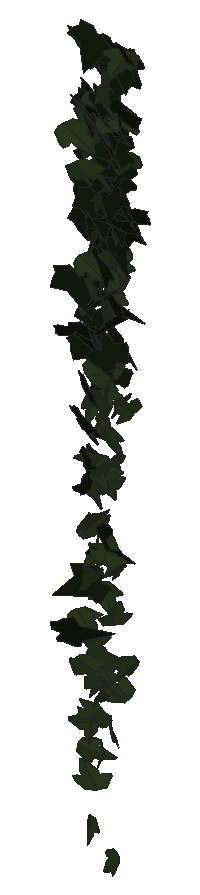
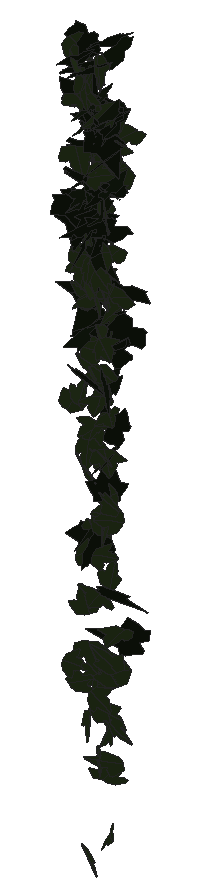
# SketchUp Ruby script. Lengths in inches.
U = 1.inch
M = Sketchup.active_model
def pt(a) = Geom::Point3d.new(a.map { |v| v * U })
def face(e, loops, mat)
  f = e.add_face(loops[0].map { |a| pt(a) })
  loops[1..].each { |l| e.add_face(l.map { |a| pt(a) }).erase! }
  f.material = f.back_material = mat if mat
  f
end
# faces: each face lists its corners as indices into pts; further lists are holes
def faces(e, pts, list, mat = nil) = list.each { |f| face(e, (f[0].is_a?(Array) ? f : [f]).map { |l| l.map { |i| pts[i] } }, mat) }
# xy, xz, yz: faces in a plane at the given z, y or x. An outline is a flat list of corners, or four numbers for a rectangle; further outlines are holes
def ring(l) = l.size == 4 ? [[l[0], l[1]], [l[2], l[1]], [l[2], l[3]], [l[0], l[3]]] : l.each_slice(2).to_a
def flat(e, list, mat, &to3) = list.each { |f| face(e, (f[0].is_a?(Array) ? f : [f]).map { |l| ring(l).map { |u, v| to3.(u, v) } }, mat) }
def xy(e, z, list, mat = nil) = flat(e, list, mat) { |x, y| [x, y, z] }
def xz(e, y, list, mat = nil) = flat(e, list, mat) { |x, z| [x, y, z] }
def yz(e, x, list, mat = nil) = flat(e, list, mat) { |y, z| [x, y, z] }
def lines(e, pts, list) = list.each { |a, b| e.add_line(pt(pts[a]), pt(pts[b])) }
# prism: a flat outline (further loops are holes) pulled along v
def prism(e, loops, v, mat = nil)
  f = face(e, loops, mat); d = Geom::Vector3d.new(v.map { |x| x * U })
  f.pushpull(f.normal.samedirection?(d) ? d.length : -d.length)
end
def box(e, o, s, mat = nil) = prism(e, [[o, [o[0] + s[0], o[1], o[2]], [o[0] + s[0], o[1] + s[1], o[2]], [o[0], o[1] + s[1], o[2]]]], [0, 0, s[2]], mat)
def at(x, y, z, deg = 0) = Geom::Transformation.translation(pt([x, y, z])) * Geom::Transformation.rotation(ORIGIN, Z_AXIS, deg.degrees)
def axes(o, x, y, z) = Geom::Transformation.new([*x, 0, *y, 0, *z, 0, *pt(o).to_a, 1])
def part(name) = M.definitions.add(name)
# library, detail: a bought-in or finely detailed component or shape, given as its bounding box
def library(name, o, s) = part(name).tap { |d| box(d.entities, o, s) }
def detail(e, o, s) = box(e.add_group.entities, o, s)
def put(e, d, t, mat = nil) = e.add_instance(d, t).tap { |i| i.material = mat if mat }
def group(e, t, mat = nil) = e.add_group.tap { |g| g.transformation = t; g.material = mat if mat }.entities
root = M.entities
M.materials.add("1026 AP 7946 SUNNY SIDE UP").color = [254, 231, 186]
M.materials.add("efeu1").color = [18, 25, 13]
M.materials.add("efeu2").color = [43, 57, 29]
c1 = part("ivyleaf_9")
p = [[1.54,2.16,1.25],[1.36,2.04,1.19],[-0.21,0.99,0.68],[-0.71,1.11,0.82],[-0.85,0.86,0.67],[-0.8,0.17,0.21],
  [-0.9,-0.01,0.1],[-0.67,-0.16,-0.02],[-0.08,-0.08,-0.05],[-0.03,-0.6,-0.4],[0.65,-0.88,-0.66],[0.83,-0.6,-0.49],
  [1.29,-0.42,-0.43],[1.8125,-0.07,-0.26],[1.21,0.44,0.15]]
faces(c1.entities,p,[[0,1,2,3,4,5,6,7,8,9,10,11,12,13,14]],"efeu1")
c2 = part("ivyleaf_10")
p = [[0,0.5,-0.03],[-0.0625,2.02,-0.43],[-0.19,2.01,-0.46],[-0.54,1.05,-0.29],[-0.52,0.625,-0.18],[-0.83,0.76,-0.28],
  [-1.16,0.64,-0.33],[-1.15,0.33,-0.24],[-0.77,-0.39,0.02],[-0.3,-0.51,0.16],[0.04,-0.48,0.23],[-0.02,2.01,-0.4375],
  [-0.06,2.01,-0.43],[0.04,-0.49,0.23],[0.67,-0.49,0.14],[1.38,0.36,-0.2],[1.375,0.51,-0.24],[0.81,0.65,-0.19],
  [0.62,0.59,-0.15],[0.6,1.09,-0.28],[0.5,1.23,-0.31]]
faces(c2.entities,p,[[0,1,2,3,4,5,6,7,8,9,10],[11,12,0,13,14,15,16,17,18,19,20]],"efeu2")
put(root,c1,axes([109.1,212.42,255.3],[-0.38815,-0.01415,0.07817],[-0.11542,-0.0364,-0.25296],[0.03792,-0.25569,0.03015]),"1026 AP 7946 SUNNY SIDE UP")
put(root,c2,axes([108.73,212.32,254.46],[0.18641,0.16961,0.10073],[0.10772,0.06995,-0.21225],[-0.28757,0.13615,-0.01421]),"1026 AP 7946 SUNNY SIDE UP")
put(root,c1,axes([108.57,212,254.15],[0.14545,0.03079,0.24435],[0.37278,0.02041,-0.09793],[-0.04766,0.25361,-0.02027]),"1026 AP 7946 SUNNY SIDE UP")
put(root,c2,axes([109.09,212.18,252.21],[0.12202,-0.07291,-0.21039],[-0.26996,0.11112,-0.10765],[0.20728,0.18765,-0.01635]),"1026 AP 7946 SUNNY SIDE UP")
put(root,c1,axes([108.75,212.23,262.23],[-0.21159,-0.16583,-0.18391],[0.21642,0.11526,-0.21765],[0.31483,-0.19068,0.02602]),"1026 AP 7946 SUNNY SIDE UP")
put(root,c2,axes([108.97,212.4,265.37],[-0.21301,-0.21353,0.03478],[-0.01266,-0.03626,-0.26041],[0.34,-0.13513,0.01209]),"1026 AP 7946 SUNNY SIDE UP")
put(root,c1,axes([108.78,211.94,261.17],[0.33078,0.13445,0.03505],[0.05691,0.00503,-0.2567],[-0.21022,0.21292,-0.01433]),"1026 AP 7946 SUNNY SIDE UP")
put(root,c2,axes([108.76,212.56,253.77],[-0.23079,-0.03638,0.15843],[0.23189,0.04469,0.15594],[-0.09019,0.20799,-0.00448]),"1026 AP 7946 SUNNY SIDE UP")
put(root,c2,axes([108.93,212.64,261.03],[-0.07149,-0.19972,0.1003],[0.04657,-0.10506,-0.20599],[0.34704,-0.02705,0.0483]),"1026 AP 7946 SUNNY SIDE UP")
put(root,c2,axes([108.87,212.35,253.33],[-0.22474,-0.15958,0.07883],[0.06279,0.06792,0.22058],[-0.27174,0.14768,-0.01422]),"1026 AP 7946 SUNNY SIDE UP")
put(root,c2,axes([108.96,212.1875,261.63],[-0.02158,0.04342,0.26265],[-0.10296,0.24615,-0.04542],[-0.39301,-0.06687,-0.00253]),"1026 AP 7946 SUNNY SIDE UP")
put(root,c1,axes([108.78,212.55,264.56],[-0.03434,-0.15433,0.22207],[0.06502,-0.21649,-0.15601],[0.41289,0.02126,0.04303]),"1026 AP 7946 SUNNY SIDE UP")
put(root,c2,axes([108.74,211.99,265.625],[0.20152,0.17099,0.17042],[0.1784,0.11998,-0.2189],[-0.32761,0.17052,-0.01437]),"1026 AP 7946 SUNNY SIDE UP")
put(root,c1,axes([108.71,212.29,267.6],[0.23756,-0.22005,0.04774],[0.02223,-0.04792,-0.27481],[0.3533,0.15098,-0.01481]),"1026 AP 7946 SUNNY SIDE UP")
put(root,c1,axes([109.13,212.34,260.06],[-0.05281,0.00819,-0.2693],[-0.35441,0.13288,0.0349],[0.20875,0.22767,-0.00889]),"1026 AP 7946 SUNNY SIDE UP")
put(root,c1,axes([109.09,212.43,265.58],[0.02018,0.23184,-0.11035],[-0.02405,-0.10768,-0.23968],[-0.40173,0.01809,0.0088]),"1026 AP 7946 SUNNY SIDE UP")
put(root,c2,axes([108.95,212.42,259.36],[0.09128,0.19116,-0.08595],[-0.03412,-0.08173,-0.20627],[-0.32688,0.06191,-0.00247]),"1026 AP 7946 SUNNY SIDE UP")
put(root,c2,axes([108.7,212.33,262.07],[0.1886,0.07448,0.21711],[0.31936,0.06243,-0.14173],[-0.14526,0.23394,-0.0297]),"1026 AP 7946 SUNNY SIDE UP")
put(root,c2,axes([108.95,212.4,249.82],[-0.01188,0.16367,-0.1463],[0.00065,-0.14302,-0.16956],[-0.34169,-0.00596,0.00477]),"1026 AP 7946 SUNNY SIDE UP")
put(root,c1,axes([108.9,212.52,266.07],[-0.06238,-0.24185,0.05581],[0.00398,-0.05664,-0.25254],[0.39017,-0.03809,0.0115]),"1026 AP 7946 SUNNY SIDE UP")
put(root,c2,axes([109.16,212.64,264.79],[0.01493,0.02693,-0.25317],[-0.21949,-0.20258,-0.02959],[-0.32112,0.13972,0.00846]),"1026 AP 7946 SUNNY SIDE UP")
put(root,c2,axes([109.1,212.65,253.02],[-0.05691,-0.17814,0.1263],[-0.02331,-0.12299,-0.18779],[0.34013,-0.03823,0.00826]),"1026 AP 7946 SUNNY SIDE UP")
put(root,c1,axes([108.83,212.65,266.18],[0.04476,-0.19415,0.17082],[0.10756,-0.15608,-0.19995],[0.38797,0.06567,0.03573]),"1026 AP 7946 SUNNY SIDE UP")
put(root,c2,axes([109.06,212.59,262.52],[-0.07905,-0.19679,0.13343],[0.04578,-0.13771,-0.20297],[0.36858,-0.0251,0.05383]),"1026 AP 7946 SUNNY SIDE UP")
put(root,c2,axes([108.8,212.52,257.36],[0.09621,-0.0488,-0.21654],[0.29213,-0.09864,0.07884],[-0.17174,-0.19514,0.01279]),"1026 AP 7946 SUNNY SIDE UP")
put(root,c1,axes([108.8,212.31,265.98],[0.21385,-0.19938,0.12808],[0.09432,-0.11078,-0.249],[0.35819,0.1482,-0.0109]),"1026 AP 7946 SUNNY SIDE UP")
put(root,c2,axes([109.01,212.57,263.93],[0.2113,-0.17684,0.10631],[0.08467,-0.08981,-0.22908],[0.31143,0.1444,-0.00985]),"1026 AP 7946 SUNNY SIDE UP")
put(root,c2,axes([109.2,212.16,261.99],[-0.04608,0.16708,-0.20215],[-0.1195,0.1841,0.17342],[0.38842,0.07646,0.02937]),"1026 AP 7946 SUNNY SIDE UP")
put(root,c2,axes([109.29,212.22,252.48],[-0.23547,-0.01911,0.18146],[-0.25383,-0.08069,-0.15078],[0.11526,-0.21675,0.03868]),"1026 AP 7946 SUNNY SIDE UP")
put(root,c2,axes([109.09,212.32,263.98],[0.08737,-0.24272,-0.07457],[0.01003,0.07402,-0.25509],[0.39753,0.05148,0.02283]),"1026 AP 7946 SUNNY SIDE UP")
put(root,c1,axes([109.18,212.59,263.11],[-0.22209,0.16617,-0.14295],[0.12399,-0.11602,-0.22497],[-0.31804,-0.16127,0.01212]),"1026 AP 7946 SUNNY SIDE UP")
put(root,c2,axes([108.96,212.32,257.51],[-0.21131,0.1088,-0.13734],[0.14687,-0.09687,-0.17818],[-0.22814,-0.16314,0.0125]),"1026 AP 7946 SUNNY SIDE UP")
put(root,c1,axes([109.04,212.3,257.48],[0.2081,0.14691,0.18135],[-0.22047,-0.10776,0.20157],[0.28398,-0.19131,0.02359]),"1026 AP 7946 SUNNY SIDE UP")
put(root,c2,axes([108.93,212.29,266.15],[-0.11879,-0.11934,-0.25786],[0.27281,0.18114,-0.14225],[0.3389,-0.18764,0.02413]),"1026 AP 7946 SUNNY SIDE UP")
put(root,c1,axes([108.78,212.24,258.97],[0.2698,-0.05383,-0.20882],[0.31725,-0.02766,0.18363],[-0.08828,-0.26389,0.02173]),"1026 AP 7946 SUNNY SIDE UP")
put(root,c2,axes([109.12,212.1875,252.06],[0.01524,-0.06895,-0.22623],[0.00945,0.2194,-0.06954],[0.36121,-0.00283,0.01136]),"1026 AP 7946 SUNNY SIDE UP")
put(root,c2,axes([109.1,212.22,255.43],[-0.06568,-0.19125,-0.12492],[-0.05705,-0.11495,0.20077],[-0.35055,0.05454,-0.00927]),"1026 AP 7946 SUNNY SIDE UP")
put(root,c1,axes([109.11,212.57,262.99],[-0.00649,0.04166,0.26319],[-0.19141,-0.22554,0.03458],[0.35878,-0.11957,0.02321]),"1026 AP 7946 SUNNY SIDE UP")
put(root,c2,axes([108.84,212.38,251.48],[-0.05062,-0.03342,-0.21837],[0.33673,0.00528,-0.03436],[0.0162,-0.21414,0.03194]),"1026 AP 7946 SUNNY SIDE UP")
put(root,c1,axes([108.8,212.18,260.78],[0.36176,-0.06074,0.10227],[0.14407,-0.0423,-0.24482],[0.11358,0.24711,-0.0152]),"1026 AP 7946 SUNNY SIDE UP")
put(root,c2,axes([109.13,212.51,267.29],[0.05166,-0.25355,-0.08],[0.01371,0.0778,-0.26229],[0.41608,0.02892,0.01857]),"1026 AP 7946 SUNNY SIDE UP")
put(root,c1,axes([109.05,212.03,259.98],[0.2795,-0.12137,-0.15354],[-0.20339,0.07335,-0.22106],[0.22242,0.2196,-0.00921]),"1026 AP 7946 SUNNY SIDE UP")
put(root,c1,axes([108.96,212.2,260.86],[0.0944,-0.22294,-0.15102],[0.00557,0.14964,-0.2341],[0.41842,0.0483,0.03719]),"1026 AP 7946 SUNNY SIDE UP")
put(root,c2,axes([108.93,212.1,264.78],[-0.27511,-0.02265,-0.2007],[0.3077,-0.00546,-0.18055],[0.0174,-0.2617,0.01959]),"1026 AP 7946 SUNNY SIDE UP")
put(root,c1,axes([108.99,212.33,264.43],[0.01334,-0.1861,-0.17521],[0.03684,0.16897,-0.18946],[0.39358,-0.00951,0.02367]),"1026 AP 7946 SUNNY SIDE UP")
put(root,c2,axes([109.1,212.01,256.7],[0.03317,-0.11659,0.25117],[-0.01919,0.24456,0.12267],[-0.42545,-0.02012,0.01405]),"1026 AP 7946 SUNNY SIDE UP")
put(root,c2,axes([109.22,212.21,258.25],[-0.25452,-0.13901,0.03922],[-0.02758,-0.03901,-0.21926],[0.22528,-0.16183,0.01746]),"1026 AP 7946 SUNNY SIDE UP")
put(root,c1,axes([108.87,212.42,263.65],[0.13034,-0.11315,-0.27031],[0.1436,0.26876,-0.08832],[0.42477,-0.05614,0.1128]),"1026 AP 7946 SUNNY SIDE UP")
put(root,c2,axes([109.23,212.14,250.91],[0.27143,0.13233,0.0767],[-0.11265,-0.02713,0.22288],[0.20985,-0.18573,0.02043]),"1026 AP 7946 SUNNY SIDE UP")
put(root,c1,axes([109.12,212.33,267.72],[-0.15424,-0.24288,0.06762],[-0.01758,-0.06765,-0.26983],[0.39578,-0.09766,0.01437]),"1026 AP 7946 SUNNY SIDE UP")
put(root,c2,axes([109.34,212.51,260.72],[-0.11031,-0.03293,0.23146],[-0.16658,-0.20346,-0.06594],[0.31615,-0.1187,0.04602]),"1026 AP 7946 SUNNY SIDE UP")
put(root,c1,axes([109.28,212.61,264.8],[-0.01787,-0.24776,-0.01424],[0.0105,-0.01273,0.25533],[-0.38993,0.01101,0.00753]),"1026 AP 7946 SUNNY SIDE UP")
put(root,c2,axes([109.2,212.375,261.09],[0.1178,-0.2316,0.0199],[-0.0008,-0.02184,-0.25078],[0.36561,0.07457,-0.00696]),"1026 AP 7946 SUNNY SIDE UP")
put(root,c1,axes([109.05,212.1875,258.3125],[0.20173,-0.19112,-0.08823],[-0.08317,0.06629,-0.23665],[0.31791,0.13862,-0.00593]),"1026 AP 7946 SUNNY SIDE UP")
put(root,c2,axes([109.27,212.22,262.15],[0.09097,-0.2529,-0.10954],[-0.05717,0.09916,-0.26638],[0.42669,0.0672,-0.01233]),"1026 AP 7946 SUNNY SIDE UP")
put(root,c2,axes([108.98,212.12,253.57],[-0.24192,-0.02677,-0.19972],[0.307,-0.0071,-0.15878],[0.01738,-0.24728,0.02471]),"1026 AP 7946 SUNNY SIDE UP")
put(root,c1,axes([109.1,212.34,261.45],[-0.04941,-0.23988,0.01052],[0.0024,-0.01188,-0.24928],[0.37761,-0.03131,0.00296]),"1026 AP 7946 SUNNY SIDE UP")
put(root,c2,axes([109.24,212.375,256.03],[-0.06052,-0.07486,0.21873],[0.00215,-0.21589,-0.07926],[0.35461,-0.01146,0.03781]),"1026 AP 7946 SUNNY SIDE UP")
put(root,c2,axes([109.21,212.33,256.63],[-0.06336,-0.1851,-0.13479],[-0.06214,-0.12404,0.19416],[-0.35,0.05553,-0.01007]),"1026 AP 7946 SUNNY SIDE UP")
put(root,c2,axes([109.03,212.49,263.04],[-0.23081,0.09377,-0.20178],[0.23223,-0.13107,-0.17895],[-0.25134,-0.20721,0.01994]),"1026 AP 7946 SUNNY SIDE UP")
put(root,c2,axes([109.28,212.31,251.52],[0.05424,-0.13626,-0.18309],[-0.06045,0.17275,-0.14376],[0.34593,0.05156,0.00359]),"1026 AP 7946 SUNNY SIDE UP")
put(root,c2,axes([109.22,212.45,259.03],[0.04481,0.11391,-0.19473],[-0.04984,-0.18717,-0.12179],[-0.3443,0.04192,-0.00771]),"1026 AP 7946 SUNNY SIDE UP")
put(root,c2,axes([109.12,212.38,256.47],[-0.13424,0.10621,0.1911],[0.19681,-0.13628,0.13939],[0.27145,0.15134,-0.00656]),"1026 AP 7946 SUNNY SIDE UP")
put(root,c1,axes([109.01,212.5625,263.98],[0.16505,-0.19349,0.11075],[0.07694,-0.097,-0.22732],[0.3403,0.11578,-0.00232]),"1026 AP 7946 SUNNY SIDE UP")
put(root,c2,axes([109.13,211.99,262.78],[0.16347,0.16372,0.14106],[0.0869,0.12539,-0.19831],[-0.32318,0.11653,0.01803]),"1026 AP 7946 SUNNY SIDE UP")
put(root,c2,axes([109.18,212.43,259.61],[0.19646,0.17664,0.02335],[0.03232,0.01196,-0.22259],[-0.27795,0.12624,-0.00938]),"1026 AP 7946 SUNNY SIDE UP")
put(root,c1,axes([108.9375,212.3,265.94],[0.29981,-0.11614,0.1605],[0.18608,-0.10488,-0.22939],[0.2434,0.22323,-0.02232]),"1026 AP 7946 SUNNY SIDE UP")
put(root,c2,axes([109.32,212.4,262],[0.09849,-0.21173,-0.07683],[-0.03496,0.06994,-0.22705],[0.35061,0.06645,-0.00106]),"1026 AP 7946 SUNNY SIDE UP")
put(root,c2,axes([109.27,211.99,256.78],[0.04966,-0.12151,0.2227],[-0.04128,0.21576,0.12974],[-0.38869,-0.03844,0.01467]),"1026 AP 7946 SUNNY SIDE UP")
put(root,c1,axes([109.18,212.44,263.78],[-0.00235,-0.13896,-0.21718],[0.01837,0.20976,-0.14184],[0.39556,-0.01057,0.0053]),"1026 AP 7946 SUNNY SIDE UP")
put(root,c1,axes([109.15,212.57,262.94],[0.13246,-0.22421,-0.04493],[-0.01752,0.04104,-0.24647],[0.35836,0.08488,0.00456]),"1026 AP 7946 SUNNY SIDE UP")
put(root,c2,axes([109.34,212.54,263.24],[0.04606,-0.23911,0.00205],[-0.00028,-0.00339,-0.24819],[0.37602,0.02929,-0.00044]),"1026 AP 7946 SUNNY SIDE UP")
put(root,c2,axes([109.25,212.1,261.02],[-0.20282,0.16408,-0.0839],[0.06941,-0.07001,-0.21526],[-0.28022,-0.1361,0.00741]),"1026 AP 7946 SUNNY SIDE UP")
put(root,c2,axes([109.33,212.15,263.5],[0.1065,-0.25129,0.07105],[0.02769,-0.06816,-0.26852],[0.40941,0.06998,-0.00032]),"1026 AP 7946 SUNNY SIDE UP")
put(root,c2,axes([109.46,212.28,263.0625],[-0.28333,0.12914,0.09329],[-0.13641,0.03235,-0.22702],[-0.20634,-0.19872,0.02198]),"1026 AP 7946 SUNNY SIDE UP")
put(root,c1,axes([109.33,212.72,267.14],[-0.16586,-0.21841,0.0802],[-0.01311,-0.08324,-0.24877],[0.36501,-0.10223,0.02751]),"1026 AP 7946 SUNNY SIDE UP")
put(root,c2,axes([109.1875,212.45,255.17],[0.32125,0.02493,0.11475],[0.17766,-0.01384,-0.21065],[-0.0239,0.23222,-0.0235]),"1026 AP 7946 SUNNY SIDE UP")
put(root,c1,axes([109.21,212.27,266.43],[0.27385,-0.16914,-0.13276],[-0.09838,0.11716,-0.24669],[0.3186,0.18156,0.03794]),"1026 AP 7946 SUNNY SIDE UP")
put(root,c2,axes([109.36,212.55,262.25],[0.07443,-0.19876,0.10275],[0.05186,-0.09574,-0.21085],[0.34662,0.057,0.00948]),"1026 AP 7946 SUNNY SIDE UP")
put(root,c2,axes([109.3,212.15,259.6875],[-0.28727,0.15853,-0.10068],[0.09738,-0.07873,-0.249],[-0.27695,-0.19211,0.01688]),"1026 AP 7946 SUNNY SIDE UP")
put(root,c1,axes([109.53,212.64,260.1875],[-0.37607,0.03084,-0.04145],[0.05775,-0.02955,-0.24734],[-0.05526,-0.24075,0.02359]),"1026 AP 7946 SUNNY SIDE UP")
put(root,c2,axes([109.4,212.16,253.01],[-0.03141,-0.15721,-0.15909],[0.02968,0.15237,-0.16236],[0.34424,-0.02748,-0.00051]),"1026 AP 7946 SUNNY SIDE UP")
put(root,c2,axes([109.55,212.12,263.14],[-0.03662,0.0151,-0.27524],[-0.16067,0.24746,0.02503],[0.38904,0.10362,-0.01557]),"1026 AP 7946 SUNNY SIDE UP")
put(root,c2,axes([109.38,212.48,262.66],[-0.04014,-0.21521,-0.07722],[0.06354,0.06873,-0.22066],[0.35202,-0.03695,0.03103]),"1026 AP 7946 SUNNY SIDE UP")
put(root,c2,axes([109.48,212.4,265.27],[0.17142,-0.2024,-0.12795],[-0.07523,0.11385,-0.23593],[0.36478,0.11859,0.01147]),"1026 AP 7946 SUNNY SIDE UP")
put(root,c1,axes([109.3,212.21,264.17],[-0.11116,-0.25942,-0.05434],[0.05221,0.04394,-0.27596],[0.4125,-0.07547,0.02028]),"1026 AP 7946 SUNNY SIDE UP")
put(root,c1,axes([109.7,212.51,265.23],[-0.30979,0.02778,0.14921],[-0.23081,-0.01647,-0.20276],[-0.0197,-0.24388,0.02923]),"1026 AP 7946 SUNNY SIDE UP")
put(root,c1,axes([109.54,212.03,262.05],[-0.06652,0.23468,-0.0414],[0.00627,-0.04147,-0.24588],[-0.37469,-0.04236,0.00324]),"1026 AP 7946 SUNNY SIDE UP")
put(root,c1,axes([109.36,212.48,263.3],[0.1666,-0.14627,-0.20563],[-0.19699,0.15449,-0.18501],[0.33434,0.16391,-0.00655]),"1026 AP 7946 SUNNY SIDE UP")
put(root,c1,axes([109.13,212.34,265.63],[0.18306,-0.2286,0.16858],[0.09976,-0.15262,-0.26495],[0.43187,0.13216,-0.01025]),"1026 AP 7946 SUNNY SIDE UP")
put(root,c1,axes([109.72,212.58,264.59],[-0.3253,0.07658,0.12127],[-0.19063,0.00688,-0.2249],[-0.11032,-0.23771,0.03103]),"1026 AP 7946 SUNNY SIDE UP")
put(root,c2,axes([109.56,212.26,253.79],[-0.34755,-0.0631,0.08747],[-0.11672,-0.04877,-0.2357],[0.11915,-0.23183,0.02426]),"1026 AP 7946 SUNNY SIDE UP")
put(root,c2,axes([109.15,212.28,260.09],[0.26976,-0.02638,-0.20707],[0.31767,0.00281,0.1774],[-0.02356,-0.26414,0.021]),"1026 AP 7946 SUNNY SIDE UP")
put(root,c2,axes([109.48,212.19,264.39],[0.01401,-0.25293,0.05225],[-0.00277,-0.05225,-0.26101],[0.40607,0.00837,-0.00359]),"1026 AP 7946 SUNNY SIDE UP")
put(root,c1,axes([109.59,212.3125,265.69],[0.02484,-0.00669,0.26555],[-0.0885,0.25197,0.01177],[-0.39573,-0.05677,0.01404]),"1026 AP 7946 SUNNY SIDE UP")
put(root,c2,axes([109.48,212.23,260.68],[-0.21809,0.19887,0.05924],[-0.07297,0.0362,-0.24896],[-0.31673,-0.14527,0.01656]),"1026 AP 7946 SUNNY SIDE UP")
put(root,c1,axes([109.32,212.59,265.86],[-0.01584,-0.24253,0.10515],[0.01675,-0.10381,-0.25027],[0.41425,-0.00508,0.01414]),"1026 AP 7946 SUNNY SIDE UP")
put(root,c2,axes([109.32,212.18,253.3125],[-0.25767,-0.09173,-0.16051],[0.23642,0.04638,-0.19142],[0.15661,-0.22094,0.02488]),"1026 AP 7946 SUNNY SIDE UP")
put(root,c2,axes([109.52,212.0625,261.95],[-0.26132,0.17708,0.05324],[-0.08604,0.01771,-0.24851],[-0.27654,-0.17284,0.02701]),"1026 AP 7946 SUNNY SIDE UP")
put(root,c2,axes([109.4,212.42,261.84],[0.02498,-0.21007,0.13645],[0.04225,0.13458,0.21543],[-0.38921,0.00112,0.03214]),"1026 AP 7946 SUNNY SIDE UP")
put(root,c2,axes([109.39,212.35,262.49],[0.31163,0.10316,0.05082],[0.06736,0.02327,-0.23004],[-0.16628,0.20276,0.00205]),"1026 AP 7946 SUNNY SIDE UP")
put(root,c2,axes([109.57,212.35,249.21],[0.1896,-0.16723,-0.0816],[-0.08376,0.05798,-0.21187],[0.27798,0.13154,-0.00819]),"1026 AP 7946 SUNNY SIDE UP")
put(root,c2,axes([109.625,212.5625,262.85],[-0.09819,-0.06747,0.22665],[-0.09845,-0.21479,-0.08727],[0.34879,-0.07962,0.03917]),"1026 AP 7946 SUNNY SIDE UP")
put(root,c1,axes([109.39,212.23,256.68],[0.25496,-0.18075,-0.13056],[-0.14798,0.08424,-0.24934],[0.31296,0.18708,-0.01153]),"1026 AP 7946 SUNNY SIDE UP")
put(root,c2,axes([109.62,212.23,252.21],[-0.18915,0.14839,0.13941],[-0.15441,0.09301,-0.19568],[-0.27444,-0.15461,0.01402]),"1026 AP 7946 SUNNY SIDE UP")
put(root,c2,axes([109.32,212.51,266.53],[0.24762,-0.07957,0.19021],[0.25372,-0.09084,-0.1822],[0.18968,0.2254,-0.00459]),"1026 AP 7946 SUNNY SIDE UP")
put(root,c1,axes([109.375,212.25,262.75],[0.03538,-0.17985,0.17311],[0.00972,-0.16929,-0.18738],[0.38799,0.02064,-0.01109]),"1026 AP 7946 SUNNY SIDE UP")
put(root,c2,axes([109.49,212.47,261.87],[0.05007,0.21115,-0.07794],[-0.02824,-0.07498,-0.22033],[-0.35219,0.03603,0.00659]),"1026 AP 7946 SUNNY SIDE UP")
put(root,c2,axes([109.52,212.45,262.5625],[-0.26164,-0.18416,-0.05742],[0.0787,0.0283,-0.25488],[0.29164,-0.17285,0.01727]),"1026 AP 7946 SUNNY SIDE UP")
put(root,c1,axes([109.62,212.12,264.42],[0.01691,0.20236,0.15323],[0.01755,0.14719,-0.20789],[-0.39345,0.01526,-0.00269]),"1026 AP 7946 SUNNY SIDE UP")
put(root,c2,axes([109.42,212.3,258.86],[-0.28001,0.07784,-0.12132],[0.15788,-0.06441,-0.19991],[-0.15684,-0.2038,0.01536]),"1026 AP 7946 SUNNY SIDE UP")
put(root,c2,axes([109.66,212.57,265.11],[-0.35185,-0.07003,0.06252],[-0.07815,-0.04439,-0.24024],[0.12346,-0.22767,0.0261]),"1026 AP 7946 SUNNY SIDE UP")
put(root,c2,axes([109.28,212.15,258.02],[0.11601,-0.09566,-0.22738],[0.32947,-0.08673,0.11064],[-0.18418,-0.2154,0.05471]),"1026 AP 7946 SUNNY SIDE UP")
put(root,c1,axes([109.53,212.09,256.27],[0.3224,0.121,-0.06467],[-0.07255,-0.0464,-0.24499],[-0.20223,0.20956,-0.01521]),"1026 AP 7946 SUNNY SIDE UP")
put(root,c1,axes([109.39,212.52,261.07],[0.24265,-0.20075,-0.00641],[-0.02333,-0.00501,-0.26043],[0.3149,0.15432,-0.01436]),"1026 AP 7946 SUNNY SIDE UP")
put(root,c2,axes([109.63,212.32,266.67],[-0.08717,-0.27447,-0.03896],[0.0193,0.0345,-0.28822],[0.4349,-0.05654,0.00498]),"1026 AP 7946 SUNNY SIDE UP")
put(root,c1,axes([109.58,212.08,261.43],[0.1209,0.1958,0.17639],[0.11249,0.15454,-0.21565],[-0.39202,0.10473,-0.00748]),"1026 AP 7946 SUNNY SIDE UP")
put(root,c1,axes([109.78,212.1,260.73],[-0.30061,-0.159,0.03155],[0.04523,0.01469,0.25615],[-0.25083,0.1932,0.00838]),"1026 AP 7946 SUNNY SIDE UP")
put(root,c2,axes([109.5625,212.04,266.92],[0.01039,-0.20836,-0.1904],[0.113,0.17872,-0.20519],[0.42184,-0.04274,0.05966]),"1026 AP 7946 SUNNY SIDE UP")
put(root,c2,axes([109.62,212.2,263.72],[-0.18943,0.20578,0.02584],[-0.04048,0.01258,-0.24504],[-0.32322,-0.12218,0.01555]),"1026 AP 7946 SUNNY SIDE UP")
put(root,c1,axes([109.59,212.32,267.69],[0.34228,-0.01779,-0.14591],[-0.22376,-0.00919,-0.22434],[0.01555,0.25948,-0.01642]),"1026 AP 7946 SUNNY SIDE UP")
put(root,c2,axes([109.76,212.43,253],[0.06646,0.08138,0.20751],[-0.16683,-0.1708,0.09324],[0.29733,-0.11403,0.00594]),"1026 AP 7946 SUNNY SIDE UP")
put(root,c2,axes([109.71,212.33,266.21],[0.40268,0.0424,-0.13869],[-0.19965,-0.05373,-0.2661],[-0.09775,0.28441,-0.02783]),"1026 AP 7946 SUNNY SIDE UP")
put(root,c2,axes([109.5,212.22,259.99],[0.05276,-0.14017,-0.20368],[0.09562,-0.18751,0.14708],[-0.36783,-0.06885,0.00902]),"1026 AP 7946 SUNNY SIDE UP")
put(root,c2,axes([109.63,212.27,254.68],[-0.14653,-0.21362,0.00667],[-0.00811,0.01063,0.23998],[-0.33601,0.0929,-0.0087]),"1026 AP 7946 SUNNY SIDE UP")
put(root,c1,axes([109.57,212.3,264.4375],[-0.06977,-0.24633,0.07701],[-0.00732,-0.0765,-0.25815],[0.40535,-0.04378,0.0086]),"1026 AP 7946 SUNNY SIDE UP")
put(root,c2,axes([109.46,212.34,257.71],[0.12341,-0.14522,-0.16822],[0.1965,-0.11147,0.16419],[-0.28069,-0.14188,0.04098]),"1026 AP 7946 SUNNY SIDE UP")
put(root,c1,axes([109.57,212.62,267.35],[-0.07727,-0.24958,-0.03294],[0.00881,0.03004,-0.26187],[0.39527,-0.04946,-0.0006]),"1026 AP 7946 SUNNY SIDE UP")
put(root,c1,axes([109.64,212.56,267.0625],[-0.17469,-0.22668,0.05463],[-0.00864,-0.05761,-0.25958],[0.36642,-0.10943,0.01992]),"1026 AP 7946 SUNNY SIDE UP")
put(root,c2,axes([109.68,212.13,258.35],[-0.12784,-0.25633,-0.09819],[0.05101,0.08817,-0.27649],[0.42619,-0.08744,0.00364]),"1026 AP 7946 SUNNY SIDE UP")
put(root,c2,axes([109.68,212.59,267.3],[0.10303,-0.2378,0.07311],[0.02327,-0.07092,-0.25448],[0.39013,0.06703,-0.00413]),"1026 AP 7946 SUNNY SIDE UP")
put(root,c2,axes([109.65,212.5,259.5],[-0.07076,-0.12991,-0.18412],[-0.01998,-0.17983,0.13748],[-0.34591,0.03697,0.02972]),"1026 AP 7946 SUNNY SIDE UP")
put(root,c1,axes([109.52,212.39,263.24],[0.09099,-0.24131,-0.00967],[-0.00991,0.00673,-0.25556],[0.37951,0.05803,-0.00435]),"1026 AP 7946 SUNNY SIDE UP")
put(root,c1,axes([109.56,212.43,263.96],[-0.02311,-0.25081,0.00595],[0.0072,-0.00748,-0.25882],[0.39448,-0.01455,0.00507]),"1026 AP 7946 SUNNY SIDE UP")
put(root,c2,axes([109.6,212.02,256.19],[0.33253,0.04651,-0.04976],[0.06679,0.03184,0.22216],[0.08196,-0.21463,0.02083]),"1026 AP 7946 SUNNY SIDE UP")
put(root,c1,axes([109.69,212.4375,263.63],[0.3249,0.021,-0.14664],[-0.21507,-0.04931,-0.21215],[-0.07082,0.24609,-0.02848]),"1026 AP 7946 SUNNY SIDE UP")
put(root,c1,axes([109.37,212.28,261.84],[0.23287,-0.08091,0.17939],[0.22763,-0.09829,-0.17401],[0.19933,0.20677,-0.01085]),"1026 AP 7946 SUNNY SIDE UP")
put(root,c1,axes([109.49,212.59,264.11],[0.11114,-0.20575,0.12467],[0.06314,-0.1154,-0.22479],[0.37093,0.08129,0.00091]),"1026 AP 7946 SUNNY SIDE UP")
put(root,c2,axes([109.68,212.38,255.91],[-0.0144,-0.01751,0.23969],[0.07825,-0.22774,-0.01696],[0.3586,0.04899,0.01333]),"1026 AP 7946 SUNNY SIDE UP")
put(root,c1,axes([109.79,212.46,263.9],[0.14935,0.17347,-0.15948],[-0.0838,-0.14761,-0.20366],[-0.35691,0.10725,-0.01892]),"1026 AP 7946 SUNNY SIDE UP")
put(root,c1,axes([109.74,212.29,266.14],[0.3305,-0.10296,0.14835],[-0.16747,0.10611,0.23797],[-0.22327,-0.232,0.04109]),"1026 AP 7946 SUNNY SIDE UP")
put(root,c1,axes([109.86,212.11,263.86],[0.12709,0.16552,-0.16066],[-0.14683,-0.12784,-0.18925],[-0.32716,0.12167,0.02252]),"1026 AP 7946 SUNNY SIDE UP")
put(root,c2,axes([109.77,212.67,253.57],[-0.011,-0.11212,0.19835],[0.0171,-0.19321,-0.11626],[0.35079,0.0059,0.01188]),"1026 AP 7946 SUNNY SIDE UP")
put(root,c2,axes([109.83,212.5625,259.36],[-0.09717,-0.13355,-0.1878],[-0.14848,-0.15557,0.15011],[-0.32177,0.11212,-0.01256]),"1026 AP 7946 SUNNY SIDE UP")
put(root,c2,axes([109.84,212.39,267.49],[-0.18854,-0.17196,0.15735],[-0.03466,-0.16391,-0.20757],[0.36101,-0.10554,0.06225]),"1026 AP 7946 SUNNY SIDE UP")
